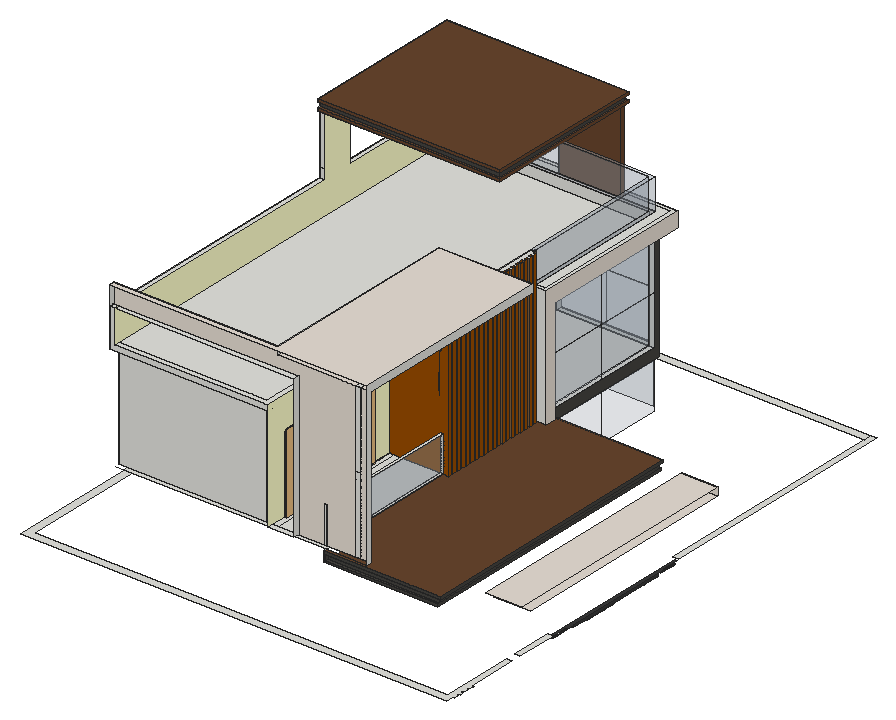
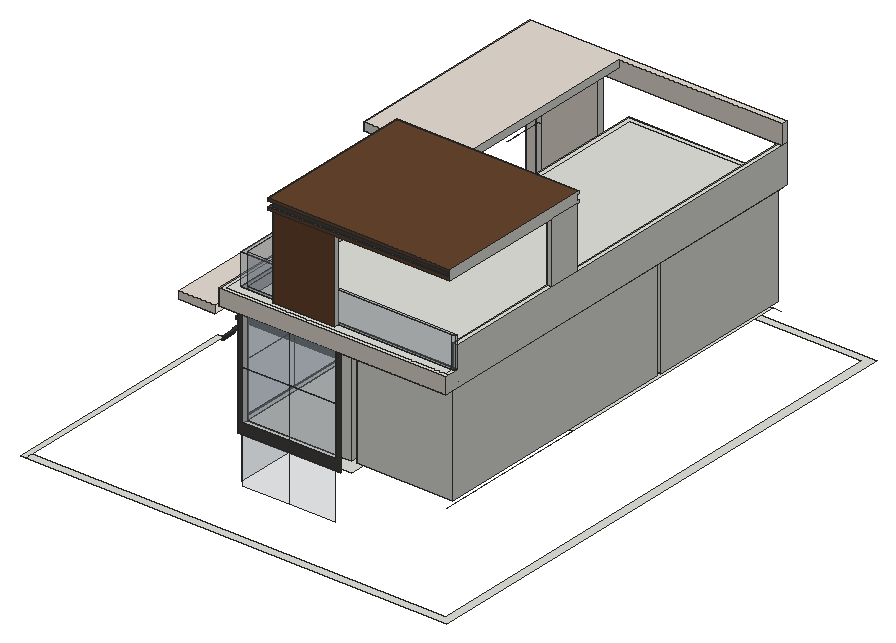
# SketchUp Ruby script. Lengths in inches.
U = 1.inch
M = Sketchup.active_model
def pt(a) = Geom::Point3d.new(a.map { |v| v * U })
def face(e, loops, mat)
  f = e.add_face(loops[0].map { |a| pt(a) })
  loops[1..].each { |l| e.add_face(l.map { |a| pt(a) }).erase! }
  f.material = f.back_material = mat if mat
  f
end
# faces: each face lists its corners as indices into pts; further lists are holes
def faces(e, pts, list, mat = nil) = list.each { |f| face(e, (f[0].is_a?(Array) ? f : [f]).map { |l| l.map { |i| pts[i] } }, mat) }
# xy, xz, yz: faces in a plane at the given z, y or x. An outline is a flat list of corners, or four numbers for a rectangle; further outlines are holes
def ring(l) = l.size == 4 ? [[l[0], l[1]], [l[2], l[1]], [l[2], l[3]], [l[0], l[3]]] : l.each_slice(2).to_a
def flat(e, list, mat, &to3) = list.each { |f| face(e, (f[0].is_a?(Array) ? f : [f]).map { |l| ring(l).map { |u, v| to3.(u, v) } }, mat) }
def xy(e, z, list, mat = nil) = flat(e, list, mat) { |x, y| [x, y, z] }
def xz(e, y, list, mat = nil) = flat(e, list, mat) { |x, z| [x, y, z] }
def yz(e, x, list, mat = nil) = flat(e, list, mat) { |y, z| [x, y, z] }
def lines(e, pts, list) = list.each { |a, b| e.add_line(pt(pts[a]), pt(pts[b])) }
# prism: a flat outline (further loops are holes) pulled along v
def prism(e, loops, v, mat = nil)
  f = face(e, loops, mat); d = Geom::Vector3d.new(v.map { |x| x * U })
  f.pushpull(f.normal.samedirection?(d) ? d.length : -d.length)
end
def box(e, o, s, mat = nil) = prism(e, [[o, [o[0] + s[0], o[1], o[2]], [o[0] + s[0], o[1] + s[1], o[2]], [o[0], o[1] + s[1], o[2]]]], [0, 0, s[2]], mat)
def at(x, y, z, deg = 0) = Geom::Transformation.translation(pt([x, y, z])) * Geom::Transformation.rotation(ORIGIN, Z_AXIS, deg.degrees)
def axes(o, x, y, z) = Geom::Transformation.new([*x, 0, *y, 0, *z, 0, *pt(o).to_a, 1])
def part(name) = M.definitions.add(name)
# library, detail: a bought-in or finely detailed component or shape, given as its bounding box
def library(name, o, s) = part(name).tap { |d| box(d.entities, o, s) }
def detail(e, o, s) = box(e.add_group.entities, o, s)
def put(e, d, t, mat = nil) = e.add_instance(d, t).tap { |i| i.material = mat if mat }
def group(e, t, mat = nil) = e.add_group.tap { |g| g.transformation = t; g.material = mat if mat }.entities
root = M.entities
M.materials.add("C07_Caramel_Shine").color = [153, 76, 0]
M.materials.add("D04_Dandelion_Burst").color = [255, 204, 50]
M.materials.add("E01_Mint_Frost").color = [255, 255, 204]
M.materials.add("Glass_Basic_01").color = [161, 173, 186]
M.materials["Glass_Basic_01"].alpha = 0.25
M.materials.add("Marble_01_1K").color = [230, 221, 211]
M.materials.add("Plywood_01_1K").color = [125, 96, 64]
M.materials.add("Wood_Planks_01_1K").color = [69, 67, 63]
M.materials.add("Wood_Veneer_15_1K").color = [103, 69, 45]
M.materials.add("[Color_007]1").color = [58, 58, 58]
M.materials.add("[Wood_Cherry_Original]1").color = [76, 43, 21]
c1 = library("porta+4",[0.2,-5.42,1.33],[46.55,4.72,83.21])
c2 = library("mesh-166",[-1553.69,-2604.3125,-42.18],[1702.88,1401.6,88.28])
c3 = part("Group30\#1")
p = [[0,0,0],[0,0,-28.26],[-0.46,0,-28.26],[3,-88.5,0],[-3,-88.5,0],[3,88.5,0],
  [3,0,0],[-3,88.5,0],[0.46,0,-28.26],[-3,0,0],[0,0,-45.75]]
lines(c3.entities,p,[[0,1],[1,2],[3,4],[5,6],[7,5],[1,8],[9,0],[0,6],[8,10],[4,9],[6,3],[2,10],
  [9,7]])
c4 = part("Rectangle Light\#1")
put(c4.entities,c3,at(0,0,0))
c5 = part("Group28\#1")
p = [[0,0,0],[0,0,-36.83],[-0.46,0,-36.83],[3,-116.25,0],[-3,-116.25,0],[3,116.25,0],
  [3,0,0],[-3,116.25,0],[0.46,0,-36.83],[-3,0,0],[0,0,-59.625]]
lines(c5.entities,p,[[0,1],[1,2],[3,4],[5,6],[7,5],[1,8],[9,0],[0,6],[8,10],[4,9],[6,3],[2,10],
  [9,7]])
c6 = part("Rectangle Light")
put(c6.entities,c5,at(0,0,0))
xy(root,54.977,[[488,324.525,490,325.45],[488,326.375,490,327.3],[488,328.225,490,329.15],[488,330.075,490,331]])
xy(root,55,[[488,201.975,492,202.95],[488,203.925,492,204.9],[488,205.875,492,206.85],[488,207.825,492,208.8],[488,209.775,492,210.75],
  [488,211.725,492,212.7],[488,213.675,492,214.65],[488,215.625,492,216.6],[488,217.575,492,218.55],[488,219.525,492,220.5],
  [488,221.475,492,222.45],[488,223.425,492,224.4],[488,225.375,492,226.35],[488,227.325,492,228.3],[488,229.275,492,230.25],
  [488,231.225,492,232.2],[488,233.175,492,234.15],[488,235.125,492,236.1],[488,237.075,492,238.05],[488,239.025,492,240],
  [488,246,490,246.975],[488,247.95,490,248.925],[488,249.9,490,250.875],[488,251.85,490,252.825],[488,253.8,490,254.775],
  [488,255.75,490,256.725],[488,257.7,490,258.675],[488,259.65,490,260.625],[488,261.6,490,262.575],[488,263.55,490,264.525],
  [488,265.5,490,266.475],[488,267.45,490,268.425],[488,269.4,490,270.375],[488,271.35,490,272.325],[488,273.3,490,274.275],
  [488,275.25,490,276.225],[488,277.2,490,278.175],[488,279.15,490,280.125],[488,281.1,490,282.075],[488,283.05,490,284.025]])
xy(root,55,[[490,201,492,201.975],[490,202.95,492,203.925],[490,204.9,492,205.875],[490,206.85,492,207.825],[490,208.8,492,209.775],
  [490,210.75,492,211.725],[490,212.7,492,213.675],[490,214.65,492,215.625],[490,216.6,492,217.575],[490,218.55,492,219.525],
  [490,220.5,492,221.475],[490,222.45,492,223.425],[490,224.4,492,225.375],[490,226.35,492,227.325],[490,228.3,492,229.275],
  [490,230.25,492,231.225],[490,232.2,492,233.175],[490,234.15,492,235.125],[490,236.1,492,237.075],[490,238.05,492,239.025],
  [490,285,492,288]],"[Color_007]1")
xy(root,58,[[488,153,490,153,490,173.5,492,173.5,492,312.5,490,312.5,490,333,488,333]],"[Color_007]1")
xy(root,60,[[0,0,492,0,492,9,494,9,494,12.75,492,12.75,492,16.5,494,16.5,494,20.25,492,20.25,492,24,494,24,494,27.75,492,27.75,492,31.5,494,31.5,494,35.25,492,35.25,492,93,486,93,486,9,9,9,9,609.138,486,609.138,486,618.138,0,618.138],[486,105,492,153],[486,333,492,618.138]])
xy(root,87,[[209.999,360,251.999,378]])
xy(root,93,[[300,297,306,339]])
xy(root,111,[[462,105,504,375]],"Marble_01_1K")
xy(root,114,[[306,54,438,57],[306,360,366,372],[180,378,300,531],[300,378,306,531],[193.503,531,300,537],
  [300,531,306,537]])
xy(root,114,[[306,63,306,360,366,360,366,372,306,372,306,375,438,375,438,63]],"Wood_Veneer_15_1K")
xy(root,117,[[309,54,438,57],[309,372,366,375],[366,372,438,375]],"Wood_Planks_01_1K")
xy(root,120,[[66,66,300,354]])
xy(root,120,[[462,93,504,375]],"Marble_01_1K")
xy(root,123,[[309,54,441,57],[438,57,441,63],[438,63,441,375],[309,372,318,375],[318,372,438,375]],"Wood_Planks_01_1K")
xy(root,126,[[240,57,270,63],[63,63,234.006,231],[240,63,246,231],[246,63,300,231],[300,63,303,231],
  [63,237,300,237,300,354,174,354,174,531,63,531],[180,360,300,531],[306,372,318,375],[300,378,306,531],[193.503,531,300,537]])
xy(root,126,[[306,54,441,54,441,375,318,375,318,360,306,360,306,356.775,309,356.775,309,353.55,306,353.55,306,350.325,309,350.325,309,347.1,306,347.1,306,343.875,309,343.875,309,340.65,306,340.65,306,337.425,309,337.425,309,334.2,306,334.2,306,330.975,309,330.975,309,327.75,306,327.75,306,324.525,309,324.525,309,321.3,306,321.3,306,318.075,309,318.075,309,314.85,306,314.85,306,311.625,309,311.625,309,308.4,306,308.4,306,305.175,309,305.175,309,301.95,306,301.95,306,298.725,309,298.725,309,295.5,306,295.5,306,292.275,309,292.275,309,289.05,306,289.05,306,285.825,309,285.825,309,282.6,306,282.6,306,279.375,309,279.375,309,276.15,306,276.15,306,272.925,309,272.925,309,269.7,306,269.7,306,266.475,309,266.475,309,263.25,306,263.25,306,260.025,309,260.025,309,256.8,306,256.8,306,253.575,309,253.575,309,250.35,306,250.35,306,247.125,309,247.125,309,243.9,306,243.9,306,240.675,309,240.675,309,237.45,306,237.45,306,234.225,309,234.225,309,231,303,231,303,63,354,63,354,57,306,57]],"Wood_Veneer_15_1K")
xy(root,129,[[234.006,84,240,204],[141.006,231,183.006,237],[210,354,252,360]])
xy(root,207,[[141.006,231,183.006,237]])
xy(root,213,[[234.006,84,240,204]])
xy(root,219,[[210,354,252,360]])
xy(root,240,[[300,378,306,531],[193.503,531,234.006,537],[234.006,531,300,537]])
xy(root,246,[[57,63,63,537],[63,63,234.006,231],[63,231,234.006,237],[63,237,63,531,174,531,174,354,234.006,354,234.006,237],[234.006,237,300,354],
  [174,354,234.006,360],[174,360,180,531],[174,360,180,531],[180,360,234.006,531],[234.006,360,300,531],
  [306,372,306,537,63,537,63,549,318,549,318,372],[63,531,234.006,537],[234.006,531,306,537],[57,537,63,549]])
xy(root,252,[[63,57,240,57,240,231,300,231,300,237,234,237,234,63,63,63],[63,63,234,63,234,237,300,237,300,531,63,531]])
xy(root,264,[[314,360,318,360,318,549,57,549,57,545,314,545],[304,360,314,364],[304,364,314,364,314,545,61,545,61,535,192.274,535,192.274,539.469,264.274,539.469,264.274,535,304,535],[57,535,61,545]])
xy(root,289.5,[[57,57,63,63],[63,57,270,63],[57,63,63,360],[57,396,63,531]])
xy(root,300,[[300,231,309,231,309,234.225,306,234.225,306,237.45,309,237.45,309,240.675,306,240.675,306,243.9,309,243.9,309,247.125,306,247.125,306,250.35,309,250.35,309,253.575,306,253.575,306,256.8,309,256.8,309,260.025,306,260.025,306,263.25,309,263.25,309,266.475,306,266.475,306,269.7,309,269.7,309,272.925,306,272.925,306,276.15,309,276.15,309,279.375,306,279.375,306,282.6,309,282.6,309,285.825,306,285.825,306,289.05,309,289.05,309,292.275,306,292.275,306,295.5,309,295.5,309,298.725,306,298.725,306,301.95,309,301.95,309,305.175,306,305.175,306,308.4,309,308.4,309,311.625,306,311.625,306,314.85,309,314.85,309,318.075,306,318.075,306,321.3,309,321.3,309,324.525,306,324.525,306,327.75,309,327.75,309,330.975,306,330.975,306,334.2,309,334.2,309,337.425,306,337.425,306,340.65,309,340.65,309,343.875,306,343.875,306,347.1,309,347.1,309,350.325,306,350.325,306,353.55,309,353.55,309,356.775,306,356.775,306,360,300,360]])
xy(root,303,[[336,63,342,295.5]])
xy(root,303,[[246.009,63,336,295.5],[342,63,354,295.5]],"Marble_01_1K")
xy(root,312,[[57,57,354,57,354,295.5,246.009,295.5,246.009,63,57,63]],"Marble_01_1K")
xy(root,360,[[57,357,63,360],[57,360,63,396],[192.274,535,264.274,539.469]])
xy(root,360,[[[87,381,243.274,511],[91,385,239.274,507]]],"D04_Dandelion_Burst")
xy(root,360,[[[63,357,63,396,57,396,57,542.469,192.274,542.469,192.274,535,264.274,535,264.274,539.469,192.274,539.469,192.274,542.469,267.274,542.469,267.274,357],[87,381,243.274,511]],[91,385,239.274,507]],"Wood_Veneer_15_1K")
xy(root,363,[[57,357,267.274,357,267.274,542.469,60,542.469,60,539.469,264.274,539.469,264.274,360,57,360]],"Wood_Veneer_15_1K")
xy(root,369,[[57,357,57,360,264.274,360,264.274,542.469,267.274,542.469,267.274,357],[60,539.469,264.274,542.469]],"Wood_Veneer_15_1K")
xy(root,372,[[57,357,267.274,542.469]],"Wood_Veneer_15_1K")
xz(root,54,[[306,114,438,114,438,117,309,117,309,123,441,123,441,126,306,126]],"Wood_Planks_01_1K")
xz(root,57,[[57,246,240,246,240,252,63,252,63,289.5,57,289.5]])
xz(root,57,[[309,117,438,123]],"Wood_Planks_01_1K")
xz(root,63,[[63,126,234.006,246],[300,126,300,167.953,303,168,303,126],[336,126,342,303]])
xz(root,63,[[270,126,270,289.5,57,289.5,57,312,246.009,312,246.009,303,336,303,336,126,303,126,303,168,300,167.953,300,126],[342,126,354,303]],"Marble_01_1K")
xz(root,84,[[234.006,129,240,213]])
xz(root,204,[[234.006,129,240,213]])
xz(root,231,[[63,126,138.006,126,138.006,210,186.006,210,186.006,126,234.006,126,234.006,246,63,246],[[138.006,126,186.006,210],[141.006,129,183.006,207]],[300,126,303,126,303,168,300,167.953]])
xz(root,231,[[240,126,300,126,300,167.953,303,168,303,126,309,126,309,300,300,300,300,252,240,252]],"C07_Caramel_Shine")
xz(root,234.225,[[306,126,309,300]],"Plywood_01_1K")
xz(root,237,[[[63,126,300,246],[141.006,129,183.006,207]]])
xz(root,237.45,[[306,126,309,300]],"Plywood_01_1K")
xz(root,240.675,[[306,126,309,300]],"Plywood_01_1K")
xz(root,243.9,[[306,126,309,300]],"Plywood_01_1K")
xz(root,247.125,[[306,126,309,300]],"Plywood_01_1K")
xz(root,250.35,[[306,126,309,300]],"Plywood_01_1K")
xz(root,253.575,[[306,126,309,300]],"Plywood_01_1K")
xz(root,256.8,[[306,126,309,300]],"Plywood_01_1K")
xz(root,260.025,[[306,126,309,300]],"Plywood_01_1K")
xz(root,263.25,[[306,126,309,300]],"Plywood_01_1K")
xz(root,266.475,[[306,126,309,300]],"Plywood_01_1K")
xz(root,269.7,[[306,126,309,300]],"Plywood_01_1K")
xz(root,272.925,[[306,126,309,300]],"Plywood_01_1K")
xz(root,276.15,[[306,126,309,300]],"Plywood_01_1K")
xz(root,279.375,[[306,126,309,300]],"Plywood_01_1K")
xz(root,282.6,[[306,126,309,300]],"Plywood_01_1K")
xz(root,285.825,[[306,126,309,300]],"Plywood_01_1K")
xz(root,289.05,[[306,126,309,300]],"Plywood_01_1K")
xz(root,292.275,[[306,126,309,300]],"Plywood_01_1K")
xz(root,295.5,[[246.009,303,354,312]])
xz(root,295.5,[[306,126,309,300]],"Plywood_01_1K")
xz(root,298.725,[[306,126,309,300]],"Plywood_01_1K")
xz(root,301.95,[[306,126,309,300]],"Plywood_01_1K")
xz(root,305.175,[[306,126,309,300]],"Plywood_01_1K")
xz(root,308.4,[[306,126,309,300]],"Plywood_01_1K")
xz(root,311.625,[[306,126,309,300]],"Plywood_01_1K")
xz(root,313.425,[[488,55,490,55.103],[488,55.103,490,55.108]])
xz(root,314.35,[[488,55,490,55.103]])
xz(root,314.85,[[306,126,309,300]],"Plywood_01_1K")
xz(root,315.275,[[488,55,490,55.098]])
xz(root,316.2,[[488,54.977,490,55],[488,55,490,55.082],[488,55.082,490,55.093]])
xz(root,317.125,[[488,54.977,490,55],[488,55,490,55.077],[488,55.077,490,55.088]])
xz(root,318.05,[[488,54.977,490,55],[488,55,490,55.072],[488,55.072,490,55.082]])
xz(root,318.075,[[306,126,309,300]],"Plywood_01_1K")
xz(root,318.975,[[488,54.977,490,55],[488,55,490,55.067],[488,55.067,490,55.077]])
xz(root,319.9,[[488,54.977,490,55],[488,55,490,55.062],[488,55.062,490,55.072]])
xz(root,320.825,[[488,54.977,490,55],[488,55,490,55.057],[488,55.057,490,55.067]])
xz(root,321.3,[[306,126,309,300]],"Plywood_01_1K")
xz(root,321.75,[[488,54.977,490,55],[488,55,490,55.051],[488,55.051,490,55.062]])
xz(root,322.675,[[488,54.977,490,55],[488,55,490,55.046],[488,55.046,490,55.057]])
xz(root,323.6,[[488,54.977,490,55],[488,55,490,55.041],[488,55.041,490,55.052]])
xz(root,324.525,[[306,126,309,300]],"Plywood_01_1K")
xz(root,327.75,[[306,126,309,300]],"Plywood_01_1K")
xz(root,330.975,[[306,126,309,300]],"Plywood_01_1K")
xz(root,334.2,[[306,126,309,300]],"Plywood_01_1K")
xz(root,337.425,[[306,126,309,300]],"Plywood_01_1K")
xz(root,340.65,[[306,126,309,300]],"Plywood_01_1K")
xz(root,343.875,[[306,126,309,300]],"Plywood_01_1K")
xz(root,347.1,[[306,126,309,300]],"Plywood_01_1K")
xz(root,350.325,[[306,126,309,300]],"Plywood_01_1K")
xz(root,353.55,[[306,126,309,300]],"Plywood_01_1K")
xz(root,354,[[[174,126,300,246],[210,129,252,219]]])
xz(root,356.775,[[306,126,309,300]],"Plywood_01_1K")
xz(root,357,[[57,360,267.274,363],[57,369,267.274,372]],"Wood_Veneer_15_1K")
xz(root,360,[[180,126,207,246],[255,126,255,222,207,222,207,246,300,246,300,126],[[207,126,255,222],[210,129,252,219]],[300,126,306,246],[306,126,318,264],
  [300,264,306,300],[57,289.5,63,300],[57,300,63,360]])
xz(root,360,[[57,363,264.274,369]],"Wood_Planks_01_1K")
xz(root,372,[[306,126,318,246]])
xz(root,372,[[309,117,438,123]],"Wood_Planks_01_1K")
xz(root,375,[[462,111,504,120]],"Marble_01_1K")
xz(root,375,[[306,114,306,126,441,126,441,123,309,123,309,117,438,117,438,114]],"Wood_Planks_01_1K")
xz(root,378,[[300,126,306,240]])
xz(root,396,[[57,289.5,63,360]])
xz(root,531,[[63,126,174,246],[180,126,193.503,126,193.503,240,300,240,300,246,180,246],[300,126,306,240],[63,252,300,264],[57,264,63,289.5]])
xz(root,531,[[193.503,126,300,240]],"Glass_Basic_01")
xz(root,535,[[192.274,264,264.274,360]],"Wood_Veneer_15_1K")
xz(root,537,[[193.503,60,246.751,114],[246.751,60,300,114],[193.503,126,246.751,183],[246.751,126,300,183],[193.503,183,246.751,240],
  [246.751,183,300,240]],"Glass_Basic_01")
xz(root,537,[[[187.503,114,306,246],[193.503,126,300,240]]],"Wood_Planks_01_1K")
xz(root,539.469,[[60,363,264.274,369]],"Wood_Planks_01_1K")
xz(root,539.469,[[192.274,264,264.274,360]],"Wood_Veneer_15_1K")
xz(root,542.469,[[57,360,57,372,267.274,372,267.274,369,60,369,60,363,267.274,363,267.274,360]],"Wood_Veneer_15_1K")
xz(root,549,[[57,246,318,264]],"Marble_01_1K")
yz(root,57,[[57,246,57,289.5,531,289.5,531,264,549,264,549,246],[57,289.5,63,312],[360,289.5,396,360],[357,360,357,363,360,363,360,369,357,369,357,372,542.469,372,542.469,360]])
yz(root,60,[[539.469,363,542.469,369]],"Wood_Veneer_15_1K")
yz(root,63,[[63,126,231,246],[237,126,531,246]])
yz(root,63,[[57,252,531,252,531,289.5,396,289.5,396,360,360,360,360,289.5,57,289.5]],"E01_Mint_Frost")
yz(root,141.006,[[231,129,237,207]])
yz(root,174,[[354,126,360,246],[360,126,531,246]])
yz(root,180,[[360,126,531,246]])
yz(root,183.006,[[231,129,237,207]])
yz(root,192.274,[[535,264,539.469,360]])
yz(root,193.503,[[531,126,537,240]])
yz(root,210,[[354,129,360,219]])
yz(root,234.006,[[[63,126,231,246],[84,129,204,213]]])
yz(root,240,[[[81,126,207,216],[84,129,204,213]]])
yz(root,240,[[57,126,81,126,81,216,207,216,207,126,231,126,231,252,57,252]],"E01_Mint_Frost")
yz(root,246.009,[[63,303,295.5,312]])
yz(root,252,[[354,129,360,219]])
yz(root,264.274,[[360,363,539.469,369]],"Wood_Planks_01_1K")
yz(root,264.274,[[535,264,539.469,360]],"Wood_Veneer_15_1K")
yz(root,267.274,[[357,360,542.469,363],[357,369,542.469,372]],"Wood_Veneer_15_1K")
yz(root,270,[[57,126,63,289.5]])
yz(root,300,[[237,126,354,246],[360,126,360,246,531,246,531,240,378,240,378,126],[531,126,537,240],[231,252,237,300],[237,252,237,300,360,300,360,264,531,264,531,252]])
yz(root,300,[[63,126,231,167.953],[378,126,531,240]],"Glass_Basic_01")
yz(root,303,[[63,126,231,168]],"Glass_Basic_01")
yz(root,306,[[54,114,57,126]])
yz(root,306,[[234.225,126,237.45,300],[240.675,126,243.9,300],[247.125,126,250.35,300],[253.575,126,256.8,300],[260.025,126,263.25,300],
  [266.475,126,269.7,300],[272.925,126,276.15,300],[279.375,126,282.6,300],[285.825,126,289.05,300],[292.275,126,295.5,300],
  [298.725,126,301.95,300],[305.175,126,308.4,300],[311.625,126,314.85,300],[318.075,126,321.3,300],[324.525,126,327.75,300],
  [330.975,126,334.2,300],[337.425,126,340.65,300],[343.875,126,347.1,300],[350.325,126,353.55,300]],"C07_Caramel_Shine")
yz(root,306,[[378,60,454.5,114],[454.5,60,531,114],[378,126,454.5,183],[454.5,126,531,183],[378,183,454.5,240],
  [454.5,183,531,240]],"Glass_Basic_01")
yz(root,306,[[356.775,126,360,300]],"Plywood_01_1K")
yz(root,306,[[375,114,454.5,114,454.5,126,378,126,378,240,531,240,531,126,454.5,126,454.5,114,537,114,537,246,372,246,372,126,375,126]],"Wood_Planks_01_1K")
yz(root,309,[[231,126,234.225,300],[237.45,126,240.675,300],[243.9,126,247.125,300],[250.35,126,253.575,300],[256.8,126,260.025,300],
  [263.25,126,266.475,300],[269.7,126,272.925,300],[276.15,126,279.375,300],[282.6,126,285.825,300],[289.05,126,292.275,300],
  [295.5,126,298.725,300],[301.95,126,305.175,300],[308.4,126,311.625,300],[314.85,126,318.075,300],[321.3,126,324.525,300],
  [327.75,126,330.975,300],[334.2,126,337.425,300],[340.65,126,343.875,300],[347.1,126,350.325,300],[353.55,126,356.775,300]],"C07_Caramel_Shine")
yz(root,309,[[54,117,57,123],[372,117,375,123]],"Wood_Planks_01_1K")
yz(root,318,[[360,126,372,126,372,246,549,246,549,264,360,264]],"Marble_01_1K")
yz(root,354,[[57,126,63,126,63,303,295.5,303,295.5,312,57,312]])
yz(root,438,[[54,114,375,117],[57,117,372,123]],"Wood_Planks_01_1K")
yz(root,441,[[54,123,375,126]],"Wood_Planks_01_1K")
yz(root,490,[[324.525,54.977,325.45,54.977,325.45,55.042,324.525,55.047],[325.45,54.977,326.375,54.977,326.375,55.037,325.45,55.042],[326.375,54.977,327.3,54.977,327.3,55.031,326.375,55.037],[327.3,54.977,328.225,54.977,328.225,55.026,327.3,55.031],[328.225,54.977,329.15,54.977,329.15,55.021,328.225,55.026],
  [329.15,54.977,330.075,54.977,330.075,55.016,329.15,55.021],[330.075,54.977,331,54.977,331,55.011,330.075,55.016],[303.5,55,312.5,55,312.5,55.114,303.5,55.164],[173.5,55.886,173.5,56,172.575,55.999,172.575,55.891],[172.575,55.891,172.575,55.999,155,56,155,55.989,156.85,55.979,157.775,55.973,163.325,55.943,165.175,55.932,170.725,55.902,171.65,55.896]])
yz(root,490,[[246,55,288,55,288,55.25,246.003,55.483]],"[Color_007]1")
yz(root,490,[[288,55,303.5,55,303.5,55.164,288,55.25]],"[Wood_Cherry_Original]1")
yz(root,492,[[303.5,55.164,303.5,58,182.5,58,182.5,55.836,198,55.75,240.003,55.517,243,55.5,246.003,55.483,288,55.25]],"[Color_007]1")
p = [[490,246,55],[490,246.003,55.483],[492,246.003,55.483],[492,246,55],[490,314.35,55.103],[490,313.425,55.108],
  [488,313.425,55.108],[488,314.35,55.103],[490,316.2,55.093],[490,315.275,55.098],[488,315.275,55.098],[488,316.2,55.093],
  [490,318.05,55.082],[490,317.125,55.088],[488,317.125,55.088],[488,318.05,55.082],[490,319.9,55.072],[490,318.975,55.077],
  [488,318.975,55.077],[488,319.9,55.072],[490,321.75,55.062],[490,320.825,55.067],[488,320.825,55.067],[488,321.75,55.062],
  [490,323.6,55.052],[490,322.675,55.057],[488,322.675,55.057],[488,323.6,55.052],[490,288,55.25],[490,303.5,55.164],
  [492,303.5,55.164],[492,288,55.25],[490,182.5,55.836],[490,198,55.75],[492,198,55.75],[492,182.5,55.836],
  [490,163.325,55.943],[490,162.4,55.948],[488,162.4,55.948],[488,163.325,55.943],[490,165.175,55.932],[490,164.25,55.9375],
  [488,164.25,55.9375],[488,165.175,55.932],[490,167.025,55.922],[490,166.1,55.927],[488,166.1,55.927],[488,167.025,55.922],
  [490,168.875,55.912],[490,167.95,55.917],[488,167.95,55.917],[488,168.875,55.912],[490,170.725,55.902],[490,169.8,55.907],
  [488,169.8,55.907],[488,170.725,55.902],[490,172.575,55.891],[490,171.65,55.896],[488,171.65,55.896],[488,172.575,55.891],
  [490,155.925,55.984],[490,155,55.989],[488,155,55.989],[488,155.925,55.984],[490,157.775,55.973],[490,156.85,55.979],
  [488,156.85,55.979],[488,157.775,55.973],[490,159.625,55.963],[490,158.7,55.968],[488,158.7,55.968],[488,159.625,55.963],
  [490,161.475,55.953],[490,160.55,55.958],[488,160.55,55.958],[488,161.475,55.953],[300,63,167.953],[303,63,168],
  [303,231,168],[300,231,167.953],[66,66,120],[57,66,120],[66,354,120],[66,360,120],
  [66,537,120],[300,66,120],[306,66,120],[252,327,126],[300,327,126],[234.006,63,246],
  [240,63,246],[300,237,246],[306,237,246],[300,354,246],[306,354,246],[300,360,120],
  [306,360,120],[57,531,252],[63,531,252],[490,173.5,55.886],[490,155.925,55.989],[490,156.85,55.99],
  [490,157.775,55.991],[490,158.7,55.991],[490,159.625,55.992],[490,160.55,55.992],[490,161.475,55.993],[490,162.4,55.993],
  [490,163.325,55.994],[490,164.25,55.994],[490,165.175,55.995],[490,166.1,55.996],[490,167.025,55.996],[490,167.95,55.997],
  [490,168.875,55.997],[490,169.8,55.998],[490,170.725,55.998],[490,171.65,55.999],[490,315.275,55.103],[490,316.2,55.103],
  [490,317.125,55.103],[490,318.05,55.103],[490,318.975,55.103],[490,319.9,55.103],[490,320.825,55.103],[490,321.75,55.103],
  [490,322.675,55.103],[490,323.6,55.103],[490,324.525,55.047],[490,324.525,55.103],[490,325.45,55.042],[490,325.45,55.103],
  [490,326.375,55.037],[490,326.375,55.103],[490,327.3,55.031],[490,327.3,55.103],[490,328.225,55.026],[490,328.225,55.103],
  [490,329.15,55.021],[490,329.15,55.103],[490,330.075,55.016],[490,330.075,55.103],[490,331,55.011],[490,331,55.103]]
faces(root,p,[[0,1,2,3],[28,29,30,31],[1,28,31,2],[32,33,34,35]],"[Color_007]1")
faces(root,p,[[4,5,6,7],[8,9,10,11],[12,13,14,15],[16,17,18,19],[20,21,22,23],[24,25,26,27],[36,37,38,39],[40,41,42,43],
  [44,45,46,47],[48,49,50,51],[52,53,54,55],[56,57,58,59],[60,61,62,63],[64,65,66,67],[68,69,70,71],[72,73,74,75],
  [76,77,78,79]])
lines(root,p,[[80,81],[82,83],[83,84],[85,86],[87,88],[89,90],[91,92],[93,94],[95,96],[97,98],[32,99],[100,60],
  [101,65],[102,64],[103,69],[104,68],[105,73],[106,72],[107,37],[108,36],[109,41],[110,40],[111,45],[112,44],
  [113,49],[114,48],[115,53],[116,52],[117,57],[9,118],[8,119],[13,120],[12,121],[17,122],[16,123],[21,124],
  [20,125],[25,126],[24,127],[128,129],[130,131],[132,133],[134,135],[136,137],[138,139],[140,141],[142,143]])
put(root,c1,axes([255.21,358.16,124.45],[-1.03118,0,0],[0,-1,0],[0,0,1.15408]))
g1 = group(root,at(240.54,174.1875,238.05))
put(g1,c2,axes([0.14,21.81,55.2],[0,0.07402,0],[0,0,0.06422],[0.03937,0,0]))
put(root,c4,axes([339,63.01,214.5],[-1,0,0],[0,0,-1],[0,-1,0]))
put(root,c6,at(339,179.25,302.99,180))
g2 = group(root,at(57,360,264),"Glass_Basic_01")
prism(g2,[[[4,175,0],[135.27,175,0],[207.27,175,0],[247,175,0],[247,4,0],[247,0,0],[243,0,0],[243,171,0],[0,171,0],[0,175,0]]],[0,0,36])
